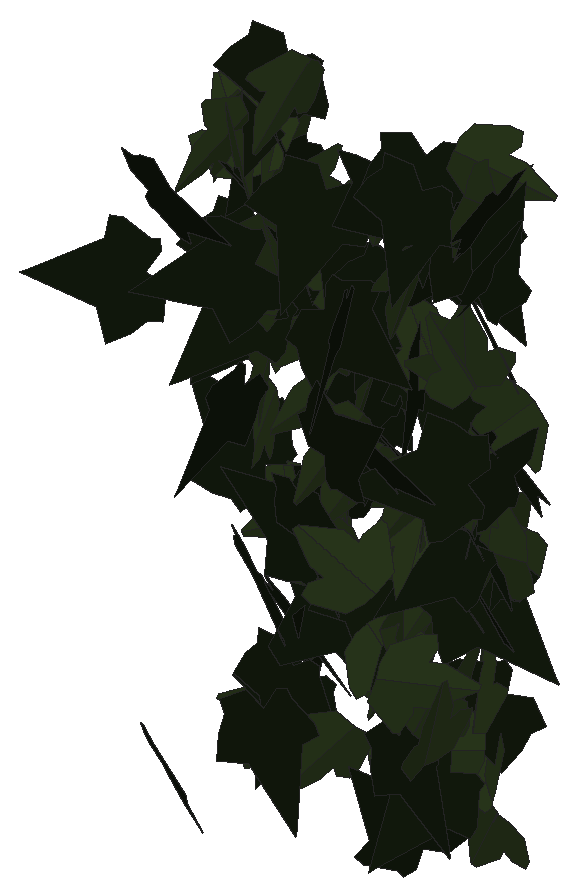
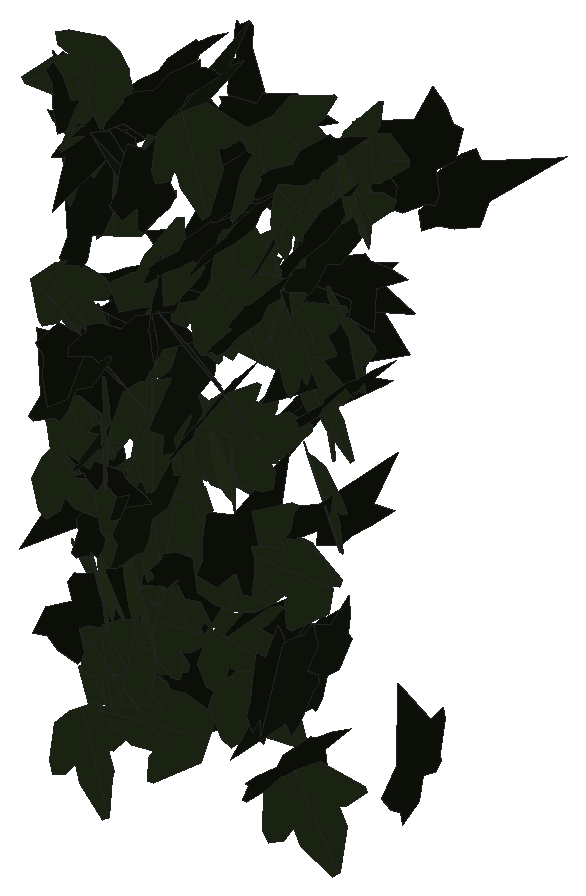
# SketchUp Ruby script. Lengths in inches.
U = 1.inch
M = Sketchup.active_model
def pt(a) = Geom::Point3d.new(a.map { |v| v * U })
def face(e, loops, mat)
  f = e.add_face(loops[0].map { |a| pt(a) })
  loops[1..].each { |l| e.add_face(l.map { |a| pt(a) }).erase! }
  f.material = f.back_material = mat if mat
  f
end
# faces: each face lists its corners as indices into pts; further lists are holes
def faces(e, pts, list, mat = nil) = list.each { |f| face(e, (f[0].is_a?(Array) ? f : [f]).map { |l| l.map { |i| pts[i] } }, mat) }
# xy, xz, yz: faces in a plane at the given z, y or x. An outline is a flat list of corners, or four numbers for a rectangle; further outlines are holes
def ring(l) = l.size == 4 ? [[l[0], l[1]], [l[2], l[1]], [l[2], l[3]], [l[0], l[3]]] : l.each_slice(2).to_a
def flat(e, list, mat, &to3) = list.each { |f| face(e, (f[0].is_a?(Array) ? f : [f]).map { |l| ring(l).map { |u, v| to3.(u, v) } }, mat) }
def xy(e, z, list, mat = nil) = flat(e, list, mat) { |x, y| [x, y, z] }
def xz(e, y, list, mat = nil) = flat(e, list, mat) { |x, z| [x, y, z] }
def yz(e, x, list, mat = nil) = flat(e, list, mat) { |y, z| [x, y, z] }
def lines(e, pts, list) = list.each { |a, b| e.add_line(pt(pts[a]), pt(pts[b])) }
# prism: a flat outline (further loops are holes) pulled along v
def prism(e, loops, v, mat = nil)
  f = face(e, loops, mat); d = Geom::Vector3d.new(v.map { |x| x * U })
  f.pushpull(f.normal.samedirection?(d) ? d.length : -d.length)
end
def box(e, o, s, mat = nil) = prism(e, [[o, [o[0] + s[0], o[1], o[2]], [o[0] + s[0], o[1] + s[1], o[2]], [o[0], o[1] + s[1], o[2]]]], [0, 0, s[2]], mat)
def at(x, y, z, deg = 0) = Geom::Transformation.translation(pt([x, y, z])) * Geom::Transformation.rotation(ORIGIN, Z_AXIS, deg.degrees)
def axes(o, x, y, z) = Geom::Transformation.new([*x, 0, *y, 0, *z, 0, *pt(o).to_a, 1])
def part(name) = M.definitions.add(name)
# library, detail: a bought-in or finely detailed component or shape, given as its bounding box
def library(name, o, s) = part(name).tap { |d| box(d.entities, o, s) }
def detail(e, o, s) = box(e.add_group.entities, o, s)
def put(e, d, t, mat = nil) = e.add_instance(d, t).tap { |i| i.material = mat if mat }
def group(e, t, mat = nil) = e.add_group.tap { |g| g.transformation = t; g.material = mat if mat }.entities
root = M.entities
M.materials.add("efeu1").color = [18, 25, 13]
M.materials.add("efeu2").color = [43, 57, 29]
c1 = part("ivyleaf_9")
p = [[1.54,2.16,1.25],[1.36,2.04,1.19],[-0.21,0.99,0.68],[-0.71,1.11,0.82],[-0.85,0.86,0.67],[-0.8,0.17,0.21],
  [-0.9,-0.01,0.1],[-0.67,-0.16,-0.02],[-0.08,-0.08,-0.05],[-0.03,-0.6,-0.4],[0.65,-0.88,-0.66],[0.83,-0.6,-0.49],
  [1.29,-0.42,-0.43],[1.8125,-0.07,-0.26],[1.21,0.44,0.15]]
faces(c1.entities,p,[[0,1,2,3,4,5,6,7,8,9,10,11,12,13,14]],"efeu1")
c2 = part("ivyleaf_10")
p = [[0,0.5,-0.03],[-0.0625,2.02,-0.43],[-0.19,2.01,-0.46],[-0.54,1.05,-0.29],[-0.52,0.625,-0.18],[-0.83,0.76,-0.28],
  [-1.16,0.64,-0.33],[-1.15,0.33,-0.24],[-0.77,-0.39,0.02],[-0.3,-0.51,0.16],[0.04,-0.48,0.23],[-0.02,2.01,-0.4375],
  [-0.06,2.01,-0.43],[0.04,-0.49,0.23],[0.67,-0.49,0.14],[1.38,0.36,-0.2],[1.375,0.51,-0.24],[0.81,0.65,-0.19],
  [0.62,0.59,-0.15],[0.6,1.09,-0.28],[0.5,1.23,-0.31]]
faces(c2.entities,p,[[0,1,2,3,4,5,6,7,8,9,10],[11,12,0,13,14,15,16,17,18,19,20]],"efeu2")
put(root,c1,axes([24.85,219.57,217.12],[0.07257,-0.47224,-0.14738],[-0.00723,0.14793,-0.47756],[0.49465,0.07145,0.01464]))
put(root,c2,axes([25.48,220.51,218.7],[0.1572,0.35375,0.31646],[-0.14851,-0.27997,0.38673],[0.45081,-0.21558,0.01705]))
put(root,c1,axes([24.94,220.61,220.12],[-0.03217,0.04607,0.49683],[0.31873,-0.38115,0.05597],[0.3839,0.32031,-0.00485]))
put(root,c1,axes([21.94,220.92,221.33],[-0.09149,-0.33367,-0.36096],[-0.0319,-0.36236,0.34304],[-0.49052,0.0858,0.04501]))
put(root,c1,axes([25,220.83,221.94],[-0.20847,0.13288,-0.43461],[0.37242,-0.22409,-0.24716],[-0.26047,-0.42676,-0.00554]))
put(root,c1,axes([21.64,221.51,222.04],[0.2449,-0.18588,0.3943],[0.30627,-0.24846,-0.30735],[0.3102,0.39207,-0.00784]))
put(root,c1,axes([22.8,221.69,219.74],[-0.11368,0.06697,-0.48228],[0.27976,-0.39635,-0.12098],[-0.39851,-0.29735,0.05264]))
put(root,c1,axes([22.82,221.83,221.33],[-0.03594,-0.25826,-0.42663],[-0.06438,-0.42175,0.26073],[-0.49453,0.07367,-0.00294]))
put(root,c1,axes([24.61,221.62,219.64],[0.23645,-0.22345,0.37968],[0.29913,-0.23492,-0.32455],[0.32343,0.38063,0.02259]))
put(root,c1,axes([21.57,221.8,214.32],[0.35903,-0.1271,-0.32395],[0.32081,-0.05945,0.37887],[-0.13483,-0.47991,0.03886]))
put(root,c2,axes([24.18,221.94,219.58],[-0.05222,-0.32041,0.38028],[0.00887,-0.38291,-0.3214],[0.49719,-0.02682,0.04567]))
put(root,c1,axes([23.63,221.83,218.46],[0.21091,-0.43924,0.11218],[0.05302,-0.09898,-0.48723],[0.45023,0.21741,0.00482]))
put(root,c1,axes([23.59,221.9375,217.98],[-0.01963,-0.49905,-0.02372],[0.00415,-0.0239,0.49941],[-0.4996,0.01941,0.00508]))
put(root,c2,axes([25.42,221.94,215.79],[0.00965,-0.49696,-0.05424],[0.0021,-0.05421,0.49705],[-0.4999,-0.00982,0.00104]))
put(root,c1,axes([24.12,221.65,221.23],[0.16564,-0.23413,-0.40957],[-0.08494,0.41219,-0.26998],[0.46406,0.15902,0.09677]))
put(root,c1,axes([23.64,222.16,222.41],[-0.36717,-0.32136,-0.10914],[0.09086,0.06184,-0.48777],[0.327,-0.37802,0.01298]))
put(root,c1,axes([24.88,222.06,215.67],[0.21484,-0.42275,-0.1585],[-0.06092,0.14679,-0.47407],[0.44736,0.22301,0.01156]))
put(root,c1,axes([25.62,222.26,219.24],[-0.31511,-0.03777,0.38637],[-0.37468,-0.10062,-0.31542],[0.10158,-0.48831,0.03511]))
put(root,c2,axes([25.02,221.79,216.67],[-0.06707,-0.15256,-0.47141],[0.35943,0.31246,-0.15225],[0.34104,-0.3593,0.06776]))
put(root,c1,axes([22.54,222.38,220.57],[-0.35125,-0.31576,0.16408],[-0.1209,-0.11095,-0.47231],[0.33468,-0.37147,0.00159]))
put(root,c2,axes([24.91,222.26,221.95],[0.04306,-0.48452,0.1157],[0.02367,-0.11401,-0.48625],[0.49758,0.04735,0.01312]))
put(root,c1,axes([25.18,222.51,215.125],[-0.31409,-0.36373,0.138],[-0.08268,-0.11091,-0.48048],[0.38015,-0.32465,0.00953]))
put(root,c1,axes([24.32,222.58,222.34],[-0.2388,-0.20372,0.38919],[0.02565,-0.44869,-0.21913],[0.43854,-0.0847,0.22475]))
put(root,c1,axes([22.89,222.51,215.72],[-0.01397,-0.48045,0.13775],[-0.00906,-0.13754,-0.48063],[0.49972,-0.01593,-0.00486]))
put(root,c1,axes([24.77,222.53,222.64],[-0.0988,-0.47595,0.1171],[0.00933,-0.12126,-0.48498],[0.49005,-0.09365,0.03284]))
put(root,c2,axes([21.92,222.59,222.5],[0.04548,-0.18705,0.46146],[0.08745,-0.45318,-0.19231],[0.49019,0.0982,-0.00851]))
put(root,c2,axes([24.95,222.53,219.02],[-0.0641,-0.33679,0.36396],[-0.02166,-0.36474,-0.34132],[0.4954,-0.05953,0.03217]))
put(root,c1,axes([24.86,222.4375,214.13],[0.18182,0.08878,0.45723],[-0.44282,-0.11922,0.19924],[0.1444,-0.47739,0.03527]))
put(root,c2,axes([25.05,222.35,216.1],[-0.35369,-0.2922,0.19881],[-0.15729,-0.12173,-0.45874],[0.31649,-0.38704,-0.00581]))
put(root,c2,axes([23.5625,222.55,215.03],[-0.18317,-0.30533,0.35103],[-0.17585,-0.30383,-0.35604],[0.43073,-0.25389,0.00393]))
put(root,c2,axes([25.41,222.51,220.52],[-0.10942,0.45569,0.17428],[0.03101,-0.17176,0.46855],[0.48689,0.11334,0.00933]))
put(root,c2,axes([25.46,222.52,220.55],[-0.39205,-0.3087,-0.03165],[-0.02229,-0.02285,0.49898],[-0.30952,0.39266,0.00415]))
put(root,c2,axes([22.61,222.35,221.58],[-0.17997,-0.44043,-0.15372],[0.05769,0.14248,-0.47578],[0.46291,-0.18899,-0.00047]))
put(root,c2,axes([24.77,222.57,218.3],[0.36781,0.32278,-0.10262],[-0.07137,-0.07423,-0.48928],[-0.3311,0.37457,-0.00853]))
put(root,c1,axes([25.38,222.67,218.16],[-0.49634,-0.01137,0.05927],[-0.05928,-0.00055,-0.49647],[0.01136,-0.49987,-0.0008]))
put(root,c2,axes([23.73,222.46,220.65],[0.00458,-0.47464,-0.15716],[-0.00644,0.1571,-0.47464],[0.49994,0.00638,-0.00467]))
put(root,c2,axes([25.14,222.83,215.32],[-0.03122,0.08987,0.49086],[-0.24231,-0.43268,0.06381],[0.43625,-0.2339,0.07057]))
put(root,c1,axes([22.15,222.78,221.0625],[-0.34576,-0.35347,-0.07424],[0.05136,0.05361,-0.49446],[0.35751,-0.34955,-0.00076]))
put(root,c2,axes([23.78,222.88,219.93],[0.06969,-0.11415,0.48178],[0.30467,-0.37362,-0.13259],[0.39028,0.31205,0.01749]))
put(root,c2,axes([22.42,222.55,219.57],[0.32751,-0.3325,-0.1794],[-0.08031,0.17073,-0.46304],[0.36917,0.33211,0.05843]))
put(root,c2,axes([21.98,222.62,222.6],[-0.20421,0.45315,-0.05434],[0.02182,-0.04976,-0.49704],[-0.45587,-0.20538,0.00055]))
put(root,c2,axes([22.76,222.98,220.0625],[-0.0478,0.25639,0.42659],[0.08705,-0.41764,0.26076],[0.49004,0.09919,-0.00471]))
put(root,c2,axes([23.21,222.37,222.16],[-0.02687,0.29903,0.39982],[-0.10191,0.38869,-0.29755],[-0.48877,-0.09748,0.04006]))
put(root,c1,axes([23.37,223.07,221.21],[-0.04007,-0.46423,0.18136],[0.0107,-0.1827,-0.4653],[0.49828,-0.03341,0.02457]))
put(root,c2,axes([21.75,222.86,222.6],[0.16171,-0.4725,0.02447],[0.00674,-0.02355,-0.4994],[0.47308,0.16184,-0.00125]))
put(root,c1,axes([24.375,223.05,220.19],[-0.05687,0.02032,-0.49634],[0.43209,-0.24445,-0.05951],[-0.24508,-0.4357,0.01024]))
put(root,c2,axes([23.68,222.98,218.57],[-0.2202,-0.35124,0.27955],[-0.12637,-0.25028,-0.414],[0.43075,-0.25297,0.02145]))
put(root,c1,axes([23.97,223.16,220.86],[-0.15419,-0.4455,0.1666],[-0.01239,-0.17131,-0.46957],[0.47547,-0.14893,0.04179]))
put(root,c2,axes([21.97,222.67,220.17],[0.23162,-0.02767,0.44225],[-0.42196,0.13856,0.22967],[-0.13527,-0.47962,0.04084]))
put(root,c1,axes([21.9,223.125,221.4375],[0.04405,-0.33715,0.3666],[0.22709,-0.31395,-0.31602],[0.44327,0.19434,0.12546]))
put(root,c1,axes([25.71,222.68,221.98],[-0.27174,0.39905,0.13007],[-0.08296,0.10082,-0.48265],[-0.41143,-0.28389,0.01142]))
put(root,c2,axes([24.78,223.09,217.49],[-0.21426,-0.3566,0.27737],[-0.06706,-0.27848,-0.40982],[0.44676,-0.21282,0.07151]))
put(root,c1,axes([24.41,223.07,222.73],[-0.06696,-0.49008,-0.07303],[0.00031,0.07366,-0.49455],[0.4955,-0.06628,-0.00956]))
put(root,c2,axes([25.1,223.07,216.36],[0.20131,-0.42004,0.18178],[0.09319,-0.15681,-0.46554],[0.4481,0.22131,0.01515]))
put(root,c2,axes([21.92,222.87,222.03],[0.37012,0.30948,0.13127],[-0.10754,-0.07598,0.48235],[0.3185,-0.38529,0.01032]))
put(root,c1,axes([25.46,222.79,221.5],[-0.35137,0.1932,0.29869],[0.24364,-0.17519,0.39993],[0.25918,0.4266,0.02897]))
put(root,c1,axes([23.95,222.95,218.89],[0.3916,-0.26191,0.16748],[0.14059,-0.09104,-0.47111],[0.27727,0.41607,0.00234]))
put(root,c1,axes([25.25,223.2,220.68],[0.09791,-0.22531,0.43549],[0.19606,-0.38905,-0.24537],[0.44942,0.21881,0.01217]))
put(root,c2,axes([24.48,223.18,218.57],[-0.05821,0.27294,-0.41487],[0.0923,-0.40448,-0.27906],[-0.48795,-0.10908,-0.00329]))
put(root,c1,axes([25.86,222.85,219.18],[-0.35718,0.28822,0.19838],[-0.1634,0.11326,-0.45877],[-0.30939,-0.39256,0.01328]))
put(root,c2,axes([25.93,222.88,218.09],[-0.10528,0.03459,0.48756],[-0.48844,0.01155,-0.10629],[-0.01861,-0.49867,0.03135]))
put(root,c1,axes([21.69,223.36,219.77],[-0.2187,-0.37182,0.25283],[-0.02659,-0.26997,-0.42001],[0.44885,-0.19715,0.09831]))
put(root,c1,axes([24.98,223.17,218.32],[0.24222,-0.39808,0.18129],[0.103,-0.1495,-0.46588],[0.42511,0.26303,0.00958]))
put(root,c1,axes([24.48,223.28,221.35],[0.04408,0.07831,0.49186],[-0.2448,-0.42661,0.08986],[0.43374,-0.24873,0.00073]))
put(root,c1,axes([21.99,223.08,217.91],[-0.27113,-0.41957,0.02116],[0.03669,0.00143,0.49865],[-0.4185,0.27195,0.03001]))
put(root,c2,axes([23.2,223.28,218.19],[0.09598,-0.28061,-0.40255],[0.15316,-0.37255,0.29622],[-0.46619,-0.18017,0.01444]))
put(root,c2,axes([24.97,223.11,215.09],[0.335,0.10336,-0.3565],[-0.33985,-0.10769,-0.35058],[-0.14926,0.4772,-0.0019]))
put(root,c2,axes([23.32,223.33,218.8],[-0.04187,-0.27073,0.41827],[-0.02406,-0.41816,-0.27306],[0.49766,-0.043,0.02199]))
put(root,c2,axes([23.98,223.34,216.06],[0.03956,-0.24547,0.4338],[0.14546,-0.41053,-0.24557],[0.47673,0.14563,0.03893]))
put(root,c1,axes([25.5,223.03,222.63],[-0.19923,0.38328,-0.2518],[0.11286,-0.22511,-0.43196],[-0.44449,-0.22896,0.00318]))
put(root,c1,axes([25.35,223.32,215.87],[-0.01206,-0.08501,-0.49257],[-0.09248,-0.48383,0.08577],[-0.49122,0.09318,-0.00406]))
put(root,c2,axes([24.34,223.08,217.05],[0.07605,-0.49395,0.01508],[0.00078,-0.01514,-0.49977],[0.49418,0.07603,-0.00153]))
put(root,c2,axes([24.5,223.01,218.62],[-0.21269,-0.4501,-0.04666],[0.01481,0.04461,-0.49779],[0.45227,-0.21313,-0.00564]))
put(root,c2,axes([23.91,223.11,222.36],[-0.17426,-0.46193,0.07911],[-0.02348,-0.07569,-0.49368],[0.46806,-0.17577,0.00468]))
put(root,c2,axes([22.35,223.29,223.03],[-0.06469,-0.39253,0.30288],[0.01623,-0.30696,-0.39435],[0.49553,-0.04119,0.05245]))
put(root,c2,axes([22.81,223.23,217.45],[-0.11223,-0.11771,0.47281],[-0.35769,-0.30956,-0.16198],[0.33085,-0.37459,-0.01472]))
put(root,c2,axes([23.91,222.86,216.27],[0.21168,0.37885,0.24833],[0.11588,0.21969,-0.43394],[-0.43791,0.24127,0.00521]))
put(root,c1,axes([21.73,223.33,216.23],[0.14785,-0.30055,0.37123],[0.16119,-0.33442,-0.33494],[0.44962,0.21871,-0.002]))
put(root,c1,axes([23.69,223.19,216.91],[-0.23489,-0.39777,-0.19132],[0.08493,0.17194,-0.46176],[0.43314,-0.24942,-0.01321]))
put(root,c1,axes([24.95,223.31,217.09],[0.14979,-0.23978,0.41239],[0.2161,-0.35124,-0.28272],[0.42528,0.26293,-0.00159]))
put(root,c1,axes([22.04,222.65,220.27],[0.19852,0.34105,0.30705],[0.12791,0.28016,-0.39389],[-0.44071,0.23494,0.02399]))
put(root,c1,axes([22.95,223.44,216.25],[-0.23091,-0.32829,0.29818],[-0.18,-0.23786,-0.40127],[0.40532,-0.29266,-0.00833]))
put(root,c2,axes([24.49,223.0625,220.1],[0.13303,0.47117,0.10149],[-0.02698,-0.09784,0.48959],[0.48122,-0.13574,-0.00061]))
put(root,c1,axes([25.13,223.01,222.01],[0.09889,-0.38649,-0.30141],[-0.03788,0.30053,-0.3978],[0.48866,0.10151,0.03016]))
put(root,c2,axes([22.02,223.11,218.65],[0.40351,-0.28887,-0.0611],[-0.04985,0.03533,-0.49625],[0.29102,0.40658,-0.00029]))
put(root,c2,axes([23.11,223.25,216.83],[-0.34129,-0.31742,-0.181],[-0.13472,-0.12092,0.46608],[-0.33966,0.36691,-0.00299]))
put(root,c2,axes([25.4375,223.3125,218.36],[-0.02643,-0.4498,0.21674],[0.05478,-0.21835,-0.44646],[0.49629,0.00015,0.06082]))
put(root,c2,axes([22.57,223.1,220.41],[-0.42095,0.25417,-0.09056],[-0.07784,0.04628,0.49173],[0.25835,0.42809,0.00061]))
put(root,c2,axes([25.29,222.99,215.81],[0.39045,-0.21796,0.22369],[-0.17655,0.14137,0.44592],[-0.25764,-0.42721,0.03343]))
put(root,c2,axes([24.75,223.08,215.45],[-0.30776,-0.38155,-0.09852],[0.06244,0.07621,-0.4902],[0.38908,-0.31403,0.00074]))
put(root,c1,axes([25.15,223.04,217.32],[0.08441,-0.30483,-0.38724],[0.13134,0.39258,-0.2804],[0.475,-0.05439,0.14635]))
put(root,c2,axes([24.21,223.08,217.26],[-0.49956,-0.00234,0.02078],[-0.02078,-0.00117,-0.49957],[0.00239,-0.49999,0.00107]))
put(root,c1,axes([22.26,223.49,214.9],[-0.15741,-0.45014,0.15033],[-0.02645,-0.14981,-0.47629],[0.47384,-0.1579,0.02335]))
put(root,c2,axes([22.64,223.54,218.92],[-0.02663,-0.05219,0.49656],[0.08078,-0.49116,-0.04729],[0.49271,0.07771,0.03459]))
put(root,c2,axes([23.15,223.39,220.58],[-0.23491,-0.34415,0.27636],[-0.05471,-0.28795,-0.40508],[0.43798,-0.22056,0.09763]))
put(root,c2,axes([22.0625,223.38,220.48],[0.00594,-0.44692,0.22411],[0.02907,-0.22343,-0.44635],[0.49912,0.01833,0.02333]))
put(root,c2,axes([25.23,222.92,222.58],[0.00017,-0.31785,-0.38597],[0.11388,0.37585,-0.30946],[0.48686,-0.0878,0.07252]))
put(root,c1,axes([25.34,223.24,219.27],[-0.12101,0.38324,-0.29746],[0.03707,-0.29838,-0.3995],[-0.48372,-0.11874,0.04379]))
put(root,c1,axes([23.35,223.5,219.0625],[0.03188,-0.46534,0.18011],[0.00685,-0.18005,-0.46641],[0.49894,0.0322,-0.0051]))
put(root,c2,axes([25.68,223.19,219.81],[0.37003,0.00275,-0.33626],[-0.33251,0.07765,-0.36525],[0.05021,0.49393,0.05929]))
put(root,c1,axes([23.96,223.09,219.61],[-0.34366,0.30268,0.2007],[-0.15746,0.12481,-0.45785],[-0.32727,-0.37789,0.00954]))
put(root,c2,axes([22.14,223.49,222.3],[0.02675,-0.3748,0.32986],[0.12999,-0.31372,-0.36699],[0.48207,0.10539,0.08066]))
put(root,c1,axes([25.07,223.4,217.69],[-0.4359,-0.16101,-0.18457],[0.17429,0.06081,-0.46468],[0.17208,-0.46944,0.00311]))
put(root,c1,axes([21.78,223.64,221.96],[-0.07951,-0.39126,0.30099],[-0.06889,-0.29309,-0.39919],[0.48881,-0.10495,-0.00729]))
put(root,c2,axes([24.46,223.34,216.62],[0.1546,-0.47439,0.0324],[0.00048,-0.03392,-0.49885],[0.4755,0.15428,-0.01003]))
put(root,c1,axes([22.48,223.56,215.55],[0.02614,0.06787,0.49468],[-0.0974,-0.48515,0.07171],[0.48973,-0.10011,-0.01214]))
put(root,c2,axes([22.01,223.26,217.29],[0.01446,0.00174,-0.49979],[0.49123,-0.09222,0.01389],[-0.09213,-0.49142,-0.00438]))
put(root,c2,axes([22.02,223.21,219.88],[0.36092,-0.17861,-0.29637],[-0.25963,0.14332,-0.40255],[0.22876,0.44447,0.0107]))
put(root,c1,axes([22.86,223.52,217.28],[0.13341,0.13837,0.46158],[-0.30535,-0.34623,0.19205],[0.37278,-0.33313,-0.00788]))
put(root,c1,axes([24.19,223.46,217.43],[0.24629,-0.34577,0.26417],[0.17241,-0.20116,-0.42404],[0.39952,0.29997,0.02014]))
put(root,c2,axes([22.04,223.375,214.57],[-0.33614,-0.30527,0.20933],[-0.15797,-0.13741,-0.45405],[0.33475,-0.37139,-0.00406]))
put(root,c2,axes([25.34,223.54,217.77],[-0.21754,-0.33431,0.30152],[-0.05573,-0.31231,-0.38647],[0.44673,-0.20175,0.09862]))
put(root,c1,axes([21.93,223.625,222.9],[-0.1814,-0.45905,0.07979],[-0.02067,-0.07761,-0.49351],[0.46548,-0.18234,0.00918]))
put(root,c1,axes([24.9,223.42,215.34],[-0.46393,0.13574,-0.12783],[0.12245,-0.03671,-0.48338],[-0.14062,-0.47982,0.00082]))
put(root,c2,axes([25.09,223.16,218.52],[0.22071,-0.32274,-0.31165],[-0.11215,0.29661,-0.38658],[0.43441,0.24055,0.05854]))
put(root,c2,axes([23.92,223.12,214.57],[0.11949,0.05804,-0.48203],[0.43845,0.20032,0.13281],[0.20854,-0.45443,-0.00302]))
put(root,c2,axes([25.16,223.27,215.3125],[0.35586,-0.20351,-0.28627],[-0.22737,0.17714,-0.40857],[0.26771,0.42096,0.03353]))
put(root,c1,axes([24.53,223.51,219.77],[-0.23272,-0.41587,-0.15132],[0.07282,0.13266,-0.47655],[0.43651,-0.24384,-0.00117]))
put(root,c2,axes([22.89,223.67,216.38],[-0.20785,-0.27087,0.36528],[0.07432,-0.41645,-0.26654],[0.44864,-0.05651,0.21338]))
put(root,c2,axes([25.02,223.26,222.9],[-0.1814,-0.04805,-0.46345],[0.46328,0.03435,-0.1849],[0.0496,-0.4965,0.03206]))
put(root,c1,axes([22.71,223.76,220.56],[-0.17609,-0.31409,0.3469],[-0.09256,-0.33995,-0.35478],[0.45872,-0.18917,0.06158]))
put(root,c1,axes([25.16,223.61,218.875],[0.09254,-0.33928,0.35542],[0.24753,-0.28023,-0.33196],[0.42446,0.2374,0.1161]))
put(root,c1,axes([22.15,223.71,221.87],[0.0474,-0.3796,0.32195],[0.02351,-0.32134,-0.38234],[0.49719,0.05138,-0.01262]))
put(root,c2,axes([25.29,223.28,214.21],[-0.41119,-0.00357,0.28444],[-0.28442,0.01412,-0.41098],[-0.0051,-0.49979,-0.01365]))
put(root,c1,axes([22.1,223.27,216.06],[0.45221,-0.18806,-0.10068],[-0.08947,0.04703,-0.48968],[0.19365,0.46089,0.00888]))
